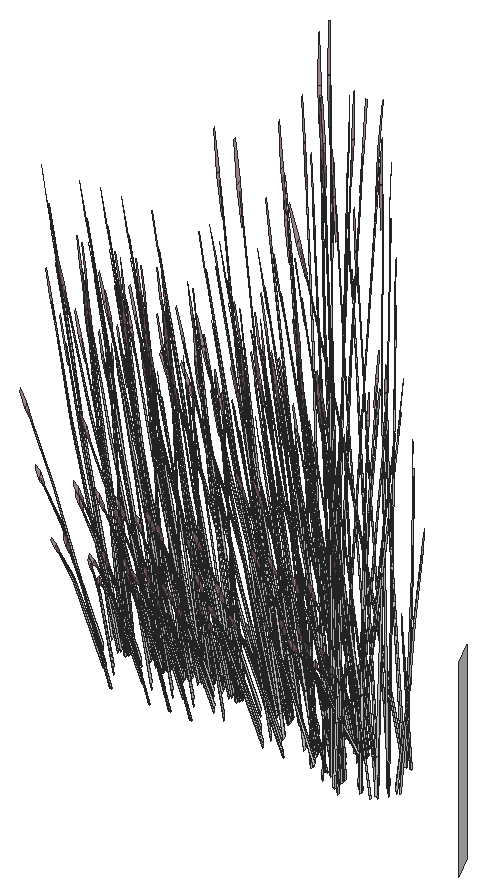
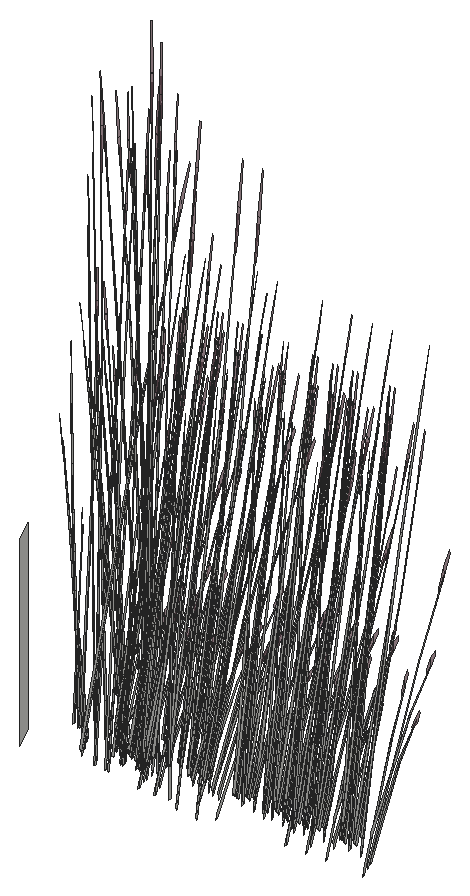
# SketchUp Ruby script. Lengths in inches.
U = 1.inch
M = Sketchup.active_model
def pt(a) = Geom::Point3d.new(a.map { |v| v * U })
def face(e, loops, mat)
  f = e.add_face(loops[0].map { |a| pt(a) })
  loops[1..].each { |l| e.add_face(l.map { |a| pt(a) }).erase! }
  f.material = f.back_material = mat if mat
  f
end
# faces: each face lists its corners as indices into pts; further lists are holes
def faces(e, pts, list, mat = nil) = list.each { |f| face(e, (f[0].is_a?(Array) ? f : [f]).map { |l| l.map { |i| pts[i] } }, mat) }
# xy, xz, yz: faces in a plane at the given z, y or x. An outline is a flat list of corners, or four numbers for a rectangle; further outlines are holes
def ring(l) = l.size == 4 ? [[l[0], l[1]], [l[2], l[1]], [l[2], l[3]], [l[0], l[3]]] : l.each_slice(2).to_a
def flat(e, list, mat, &to3) = list.each { |f| face(e, (f[0].is_a?(Array) ? f : [f]).map { |l| ring(l).map { |u, v| to3.(u, v) } }, mat) }
def xy(e, z, list, mat = nil) = flat(e, list, mat) { |x, y| [x, y, z] }
def xz(e, y, list, mat = nil) = flat(e, list, mat) { |x, z| [x, y, z] }
def yz(e, x, list, mat = nil) = flat(e, list, mat) { |y, z| [x, y, z] }
def lines(e, pts, list) = list.each { |a, b| e.add_line(pt(pts[a]), pt(pts[b])) }
# prism: a flat outline (further loops are holes) pulled along v
def prism(e, loops, v, mat = nil)
  f = face(e, loops, mat); d = Geom::Vector3d.new(v.map { |x| x * U })
  f.pushpull(f.normal.samedirection?(d) ? d.length : -d.length)
end
def box(e, o, s, mat = nil) = prism(e, [[o, [o[0] + s[0], o[1], o[2]], [o[0] + s[0], o[1] + s[1], o[2]], [o[0], o[1] + s[1], o[2]]]], [0, 0, s[2]], mat)
def at(x, y, z, deg = 0) = Geom::Transformation.translation(pt([x, y, z])) * Geom::Transformation.rotation(ORIGIN, Z_AXIS, deg.degrees)
def axes(o, x, y, z) = Geom::Transformation.new([*x, 0, *y, 0, *z, 0, *pt(o).to_a, 1])
def part(name) = M.definitions.add(name)
# library, detail: a bought-in or finely detailed component or shape, given as its bounding box
def library(name, o, s) = part(name).tap { |d| box(d.entities, o, s) }
def detail(e, o, s) = box(e.add_group.entities, o, s)
def put(e, d, t, mat = nil) = e.add_instance(d, t).tap { |i| i.material = mat if mat }
def group(e, t, mat = nil) = e.add_group.tap { |g| g.transformation = t; g.material = mat if mat }.entities
root = M.entities
M.materials.add("LightPink_Translucent").color = [144, 107, 117]
M.materials["LightPink_Translucent"].alpha = 0.75
c1 = part("blade")
p = [[2.15,0.21,22],[0,0.17,0],[0.09,0.45,0],[2.18,0.31,22],[2.29,0.31,22],[0.38,0.45,0],
  [2.48,0.24,33],[2.49,0.24,33],[2.48,0.22,33]]
faces(c1.entities,p,[[0,1,2,3],[4,5,2,3],[6,3,4,7],[8,0,3,6]])
c2 = part("seeds")
p = [[0.3,-0.1,1.38],[-0.01,-0.03,1.59],[-0.01,-0.03,0.03],[0.14,-0.07,-0.07],[0.29,-0.03,3],[0.15,0.01,3.11]]
faces(c2.entities,p,[[0,1,2,3],[1,0,4,5]],"LightPink_Translucent")
c3 = part("blade with seeds")
put(c3.entities,c1,at(0,0,0))
put(c3.entities,c2,axes([2.4,0.25,30.99],[1.5799,-0.05474,1.17369],[-0.12525,1.92788,0.29478],[-0.07173,-0.02425,1.56792]))
p = [[372.76,351.04,618],[373.98,348.58,618],[373.98,348.58,636],[372.76,351.04,636]]
faces(root,p,[[0,1,2,3]])
put(root,c3,axes([358.76,353.51,622.98],[-0.16845,-0.3792,-0.71045],[0.34676,-0.21133,0.08574],[-0.03939,-0.18322,1.00501]))
put(root,c3,axes([337.4375,352.92,620.59],[-0.02137,0.15256,1.43002],[-0.31245,0.12771,-0.30754],[-0.07303,-0.19719,0.61141]))
put(root,c3,axes([360.3,353.52,622.98],[-0.16845,-0.3792,-0.71045],[0.34676,-0.21133,0.08574],[-0.03939,-0.18322,1.00501]))
put(root,c3,axes([364.08,350.79,620.13],[-0.2439,0.26754,-0.03893],[-0.22348,-0.29302,-0.17649],[-0.01573,-0.08303,0.58215]))
put(root,c3,axes([342.99,352.94,620.59],[-0.02137,0.15256,1.43002],[-0.31245,0.12771,-0.30754],[-0.07303,-0.19719,0.61141]))
put(root,c3,axes([353.66,352.8,622.68],[-0.34695,-0.11691,-0.51099],[0.11892,-0.40083,-0.3958],[-0.03181,-0.16138,0.97773]))
put(root,c3,axes([353.87,351.8,620.77],[0.04528,0.27194,1.1486],[-0.25117,-0.15062,0.84392],[0.02703,-0.13924,0.25299]))
put(root,c3,axes([341.92,352.51,619.49],[-0.0592,0.0168,1.76342],[-0.32738,-0.18913,-0.26939],[0.00549,-0.15776,0.30037]))
put(root,c3,axes([345.83,352.52,619.49],[-0.0592,0.0168,1.76342],[-0.32738,-0.18913,-0.26939],[0.00549,-0.15776,0.30037]))
put(root,c3,axes([360.47,351.21,620.43],[0.39767,0.22603,0.24065],[-0.19139,0.46966,0.50002],[0,-0.10827,1.60543]))
put(root,c3,axes([357.66,353,620.59],[-0.02137,0.15256,1.43002],[-0.31245,0.12771,-0.30754],[-0.07303,-0.19719,0.61141]))
put(root,c3,axes([350.43,352.81,622.72],[-0.00341,-0.09282,1.74944],[-0.28775,-0.26825,-0.27667],[0.04449,-0.16261,0.14031]))
put(root,c3,axes([349.22,352.79,622.53],[0.1064,-0.35863,-0.35414],[0.31043,0.1046,0.4572],[-0.02846,-0.14439,0.87481]))
put(root,c3,axes([360.32,351.84,620.4375],[0.09355,-0.55261,-0.23429],[0.44354,0.09633,0.51271],[-0.0775,-0.07631,1.5644]))
put(root,c3,axes([349.46,353.26,621.875],[-0.06572,0.16029,1.71376],[-0.27569,-0.33172,0.13857],[0.12437,-0.20675,0.73262]))
put(root,c3,axes([359.2,353.01,620.59],[-0.02137,0.15256,1.43002],[-0.31245,0.12771,-0.30754],[-0.07303,-0.19719,0.61141]))
put(root,c3,axes([350.35,352.47,622.71],[-0.03584,0.03562,1.77383],[-0.35118,-0.12018,-0.16761],[-0.01271,-0.15545,0.31391]))
put(root,c3,axes([355.12,352.28,623.09],[0.39316,-0.11987,0.53763],[0.06823,0.47021,0.4433],[-0.09247,-0.13858,1.11249]))
put(root,c3,axes([354.41,353.1,622.68],[-0.25266,-0.31335,-0.51099],[0.2669,-0.27442,-0.3958],[0.03844,-0.15921,0.97773]))
put(root,c3,axes([338.24,352.59,619.49],[-0.0592,0.0168,1.76342],[-0.32738,-0.18913,-0.26939],[0.00549,-0.15776,0.30037]))
put(root,c3,axes([359.33,350.21,622.68],[-0.25628,0.30892,-0.51099],[-0.22444,-0.32634,-0.3958],[-0.13021,-0.047,0.97773]))
put(root,c3,axes([343.79,352.61,619.49],[-0.0592,0.0168,1.76342],[-0.32738,-0.18913,-0.26939],[0.00549,-0.15776,0.30037]))
put(root,c3,axes([362.875,350.92,622.72],[-0.07594,-0.00329,1.74944],[-0.24177,0.32918,-0.27667],[-0.129,-0.06726,0.14031]))
put(root,c3,axes([365.74,352.56,623.03],[-0.32648,-0.25715,-0.1216],[0.18809,-0.3724,-0.67495],[0.09224,-0.12945,1.02557]))
put(root,c3,axes([356.01,352.36,622.73],[0.34777,0.12192,0.48003],[-0.11892,0.40083,0.3958],[-0.0209,-0.15763,0.9933]))
put(root,c3,axes([359.52,350.07,623.05],[0.20082,0.29199,0.35414],[-0.2293,0.2764,-0.4572],[-0.1165,-0.04206,0.87481]))
put(root,c3,axes([358.47,352.66,619.49],[-0.0592,0.0168,1.76342],[-0.32738,-0.18913,-0.26939],[0.00549,-0.15776,0.30037]))
put(root,c3,axes([342.91,353.72,622.98],[0.00918,-0.43138,-0.71045],[0.38672,0.02897,0.08574],[0.04081,-0.18275,1.00501]))
put(root,c3,axes([356.11,352.51,623.03],[-0.34538,0.21713,-0.1216],[-0.16972,-0.38536,-0.67495],[-0.04557,-0.16239,1.02557]))
put(root,c3,axes([353.04,351.56,622.71],[-0.00658,0.0559,1.77383],[-0.32474,0.20287,-0.16761],[-0.09556,-0.1037,0.31391]))
put(root,c3,axes([360.01,352.68,619.49],[-0.0592,0.0168,1.76342],[-0.32738,-0.18913,-0.26939],[0.00549,-0.15776,0.30037]))
put(root,c3,axes([346.83,353.73,622.98],[0.00918,-0.43138,-0.71045],[0.38672,0.02897,0.08574],[0.04081,-0.18275,1.00501]))
put(root,c3,axes([356.83,352.99,623.03],[-0.3879,-0.02311,-0.1216],[0.0106,-0.43749,-0.67495],[0.02694,-0.1685,1.02557]))
put(root,c3,axes([358.75,350.62,620.77],[0.22533,-0.03337,1.1486],[-0.14293,0.29403,0.84392],[-0.11135,-0.04411,0.25299]))
put(root,c3,axes([356.8,352.71,622.53],[0.23881,-0.24554,-0.35414],[0.22606,0.28036,0.4572],[0.0344,-0.14245,0.87481]))
put(root,c3,axes([354.74,351.85,620.77],[0.18411,0.16231,1.1486],[-0.26813,0.09757,0.84392],[-0.05737,-0.12474,0.25299]))
put(root,c3,axes([356.1,352.33,622.73],[0.26007,-0.1585,0.0643],[0.12729,0.28902,0.50621],[-0.02512,-0.1274,0.77189]))
put(root,c3,axes([349.0625,353.03,622.68],[-0.34695,-0.11691,-0.51099],[0.11892,-0.40083,-0.3958],[-0.03181,-0.16138,0.97773]))
put(root,c3,axes([355.18,352.71,622.98],[-0.30095,-0.22541,-0.71045],[0.21388,-0.395,0.08574],[-0.10904,-0.13459,1.00501]))
put(root,c3,axes([349.28,352.03,620.77],[0.04528,0.27194,1.1486],[-0.25117,-0.15062,0.84392],[0.02703,-0.13924,0.25299]))
put(root,c3,axes([339.23,353.8,622.98],[0.00918,-0.43138,-0.71045],[0.38672,0.02897,0.08574],[0.04081,-0.18275,1.00501]))
put(root,c3,axes([344.78,353.82,622.98],[0.00918,-0.43138,-0.71045],[0.38672,0.02897,0.08574],[0.04081,-0.18275,1.00501]))
put(root,c3,axes([355.08,352.41,622.53],[-0.05451,-0.37564,-0.35414],[0.31161,-0.09919,0.4572],[-0.0837,-0.10765,0.87481]))
put(root,c3,axes([343.45,353.05,622.72],[-0.00341,-0.09282,1.74944],[-0.28775,-0.26825,-0.27667],[0.04449,-0.16261,0.14031]))
put(root,c3,axes([342.24,353.03,622.53],[0.1064,-0.35863,-0.35414],[0.31043,0.1046,0.4572],[-0.02846,-0.14439,0.87481]))
put(root,c3,axes([342.48,353.5,621.875],[-0.06572,0.16029,1.71376],[-0.27569,-0.33172,0.13857],[0.12437,-0.20675,0.73262]))
put(root,c3,axes([347.37,353.06,622.72],[-0.00341,-0.09282,1.74944],[-0.28775,-0.26825,-0.27667],[0.04449,-0.16261,0.14031]))
put(root,c3,axes([343.37,352.71,622.71],[-0.03584,0.03562,1.77383],[-0.35118,-0.12018,-0.16761],[-0.01271,-0.15545,0.31391]))
put(root,c3,axes([346.16,353.04,622.53],[0.1064,-0.35863,-0.35414],[0.31043,0.1046,0.4572],[-0.02846,-0.14439,0.87481]))
put(root,c3,axes([346.39,353.51,621.875],[-0.06572,0.16029,1.71376],[-0.27569,-0.33172,0.13857],[0.12437,-0.20675,0.73262]))
put(root,c3,axes([347.29,352.72,622.71],[-0.03584,0.03562,1.77383],[-0.35118,-0.12018,-0.16761],[-0.01271,-0.15545,0.31391]))
put(root,c3,axes([349.8125,353.34,622.68],[-0.25266,-0.31335,-0.51099],[0.2669,-0.27442,-0.3958],[0.03844,-0.15921,0.97773]))
put(root,c3,axes([359.46,353.875,622.98],[0.00918,-0.43138,-0.71045],[0.38672,0.02897,0.08574],[0.04081,-0.18275,1.00501]))
put(root,c3,axes([360.34,350.89,620.72],[-0.38326,0.02879,0.44739],[-0.03466,-0.47788,-0.21531],[0.06861,-0.04843,1.43643]))
put(root,c3,axes([361,353.89,622.98],[0.00918,-0.43138,-0.71045],[0.38672,0.02897,0.08574],[0.04081,-0.18275,1.00501]))
put(root,c3,axes([352.96,352.55,623.09],[0.39316,-0.11987,0.53763],[0.06823,0.47021,0.4433],[-0.09247,-0.13858,1.11249]))
put(root,c3,axes([364.39,353.96,621.33],[0.305,0.18805,1.51261],[-0.29879,0.40513,0.59816],[-0.13384,-0.24012,1.26806]))
put(root,c3,axes([359.46,349.89,623.03],[-0.0189,0.47427,-0.1216],[-0.35781,-0.01296,-0.67495],[-0.13781,-0.03295,1.02557]))
put(root,c3,axes([359.35,351.24,620.48],[0,0.46636,0.49651],[-0.39487,0,0],[0,-0.10622,1.57504]))
put(root,c3,axes([339.77,353.125,622.72],[-0.00341,-0.09282,1.74944],[-0.28775,-0.26825,-0.27667],[0.04449,-0.16261,0.14031]))
put(root,c3,axes([338.5625,353.11,622.53],[0.1064,-0.35863,-0.35414],[0.31043,0.1046,0.4572],[-0.02846,-0.14439,0.87481]))
put(root,c3,axes([338.8,353.58,621.875],[-0.06572,0.16029,1.71376],[-0.27569,-0.33172,0.13857],[0.12437,-0.20675,0.73262]))
put(root,c3,axes([339.69,352.79,622.71],[-0.03584,0.03562,1.77383],[-0.35118,-0.12018,-0.16761],[-0.01271,-0.15545,0.31391]))
put(root,c3,axes([345.32,353.15,622.72],[-0.00341,-0.09282,1.74944],[-0.28775,-0.26825,-0.27667],[0.04449,-0.16261,0.14031]))
put(root,c3,axes([344.11,353.13,622.53],[0.1064,-0.35863,-0.35414],[0.31043,0.1046,0.4572],[-0.02846,-0.14439,0.87481]))
put(root,c3,axes([344.35,353.6,621.875],[-0.06572,0.16029,1.71376],[-0.27569,-0.33172,0.13857],[0.12437,-0.20675,0.73262]))
put(root,c3,axes([345.24,352.82,622.71],[-0.03584,0.03562,1.77383],[-0.35118,-0.12018,-0.16761],[-0.01271,-0.15545,0.31391]))
put(root,c3,axes([363.75,351.42,623.05],[0.05451,0.37564,0.35414],[-0.31161,0.09919,-0.4572],[-0.0837,-0.10765,0.87481]))
put(root,c3,axes([348.44,351.79,622.71],[-0.00658,0.0559,1.77383],[-0.32474,0.20287,-0.16761],[-0.09556,-0.1037,0.31391]))
put(root,c3,axes([353.85,352.64,622.73],[0.34777,0.12192,0.48003],[-0.11892,0.40083,0.3958],[-0.0209,-0.15763,0.9933]))
put(root,c3,axes([362.14,351.71,623.03],[-0.17758,-0.42229,-0.1216],[0.31518,-0.20752,-0.67495],[0.13282,-0.05572,1.02557]))
put(root,c3,axes([362.125,351.34,622.68],[0.09562,-0.42421,-0.51099],[0.32782,0.1454,-0.3958],[0.13199,-0.0389,0.97773]))
put(root,c3,axes([362.8,352.66,620.02],[0,-0.46636,-0.49651],[0.39487,0,0],[0,-0.10622,1.57504]))
put(root,c3,axes([363.9,351.28,620.02],[0.33032,-0.23318,-0.49651],[0.19744,0.41812,0],[0.07523,-0.05311,1.57504]))
put(root,c3,axes([360,353.2,622.72],[-0.00341,-0.09282,1.74944],[-0.28775,-0.26825,-0.27667],[0.04449,-0.16261,0.14031]))
put(root,c3,axes([361.61,349.62,620.375],[0.22066,-0.46731,0],[0.36918,0.26061,-0.51607],[0.08408,0.05936,1.63711]))
put(root,c3,axes([358.79,353.18,622.53],[0.1064,-0.35863,-0.35414],[0.31043,0.1046,0.4572],[-0.02846,-0.14439,0.87481]))
put(root,c3,axes([353.95,352.78,623.03],[-0.34538,0.21713,-0.1216],[-0.16972,-0.38536,-0.67495],[-0.04557,-0.16239,1.02557]))
put(root,c3,axes([359.03,353.66,621.875],[-0.06572,0.16029,1.71376],[-0.27569,-0.33172,0.13857],[0.12437,-0.20675,0.73262]))
put(root,c3,axes([359.92,352.87,622.71],[-0.03584,0.03562,1.77383],[-0.35118,-0.12018,-0.16761],[-0.01271,-0.15545,0.31391]))
put(root,c3,axes([361.54,353.21,622.72],[-0.00341,-0.09282,1.74944],[-0.28775,-0.26825,-0.27667],[0.04449,-0.16261,0.14031]))
put(root,c3,axes([360.33,353.2,622.53],[0.1064,-0.35863,-0.35414],[0.31043,0.1046,0.4572],[-0.02846,-0.14439,0.87481]))
put(root,c3,axes([360.5625,353.67,621.875],[-0.06572,0.16029,1.71376],[-0.27569,-0.33172,0.13857],[0.12437,-0.20675,0.73262]))
put(root,c3,axes([365.86,352.09,620.59],[-0.12609,-0.01381,1.43002],[-0.12917,-0.37055,-0.30754],[0.1549,-0.10482,0.61141]))
put(root,c3,axes([362.82,351.66,623.09],[0.29147,-0.34417,0.53763],[0.25138,0.3655,0.4433],[-0.13675,-0.06349,1.11249]))
put(root,c3,axes([361.46,352.88,622.71],[-0.03584,0.03562,1.77383],[-0.35118,-0.12018,-0.16761],[-0.01271,-0.15545,0.31391]))
put(root,c3,axes([354.67,353.27,623.03],[-0.3879,-0.02311,-0.1216],[0.0106,-0.43749,-0.67495],[0.02694,-0.1685,1.02557]))
put(root,c3,axes([342.08,353.27,622.68],[-0.34695,-0.11691,-0.51099],[0.11892,-0.40083,-0.3958],[-0.03181,-0.16138,0.97773]))
put(root,c3,axes([366.55,352.44,622.71],[-0.0461,-0.00354,1.77383],[-0.19143,-0.37951,-0.16761],[0.07688,-0.12478,0.31391]))
put(root,c3,axes([359.01,350.54,621.875],[0.14639,-0.01056,1.71376],[-0.09712,0.45778,0.13857],[-0.20862,-0.02831,0.73262]))
put(root,c3,axes([342.3,352.27,620.77],[0.04528,0.27194,1.1486],[-0.25117,-0.15062,0.84392],[0.02703,-0.13924,0.25299]))
put(root,c3,axes([346,353.28,622.68],[-0.34695,-0.11691,-0.51099],[0.11892,-0.40083,-0.3958],[-0.03181,-0.16138,0.97773]))
put(root,c3,axes([354.64,352.99,622.53],[0.23881,-0.24554,-0.35414],[0.22606,0.28036,0.4572],[0.0344,-0.14245,0.87481]))
put(root,c3,axes([360.29,351.62,620.21],[-0.21202,-0.39143,-0.44739],[0.32115,-0.27564,0.21531],[-0.06861,-0.04843,1.43643]))
put(root,c3,axes([360.33,351.0625,620.36],[0.15345,0.52148,0.45755],[-0.43845,0.18134,0.17955],[0.00536,-0.09582,1.58856]))
put(root,c3,axes([352.58,352.125,620.77],[0.18411,0.16231,1.1486],[-0.26813,0.09757,0.84392],[-0.05737,-0.12474,0.25299]))
put(root,c3,axes([346.21,352.28,620.77],[0.04528,0.27194,1.1486],[-0.25117,-0.15062,0.84392],[0.02703,-0.13924,0.25299]))
put(root,c3,axes([353.95,352.61,622.73],[0.26007,-0.1585,0.0643],[0.12729,0.28902,0.50621],[-0.02512,-0.1274,0.77189]))
put(root,c3,axes([353.02,352.98,622.98],[-0.30095,-0.22541,-0.71045],[0.21388,-0.395,0.08574],[-0.10904,-0.13459,1.00501]))
put(root,c3,axes([352.92,352.69,622.53],[-0.05451,-0.37564,-0.35414],[0.31161,-0.09919,0.4572],[-0.0837,-0.10765,0.87481]))
put(root,c3,axes([338.4,353.35,622.68],[-0.34695,-0.11691,-0.51099],[0.11892,-0.40083,-0.3958],[-0.03181,-0.16138,0.97773]))
put(root,c3,axes([342.83,353.58,622.68],[-0.25266,-0.31335,-0.51099],[0.2669,-0.27442,-0.3958],[0.03844,-0.15921,0.97773]))
put(root,c3,axes([338.62,352.35,620.77],[0.04528,0.27194,1.1486],[-0.25117,-0.15062,0.84392],[0.02703,-0.13924,0.25299]))
put(root,c3,axes([346.75,353.59,622.68],[-0.25266,-0.31335,-0.51099],[0.2669,-0.27442,-0.3958],[0.03844,-0.15921,0.97773]))
put(root,c3,axes([348.37,352.78,623.09],[0.39316,-0.11987,0.53763],[0.06823,0.47021,0.4433],[-0.09247,-0.13858,1.11249]))
put(root,c3,axes([343.95,353.375,622.68],[-0.34695,-0.11691,-0.51099],[0.11892,-0.40083,-0.3958],[-0.03181,-0.16138,0.97773]))
put(root,c3,axes([344.17,352.37,620.77],[0.04528,0.27194,1.1486],[-0.25117,-0.15062,0.84392],[0.02703,-0.13924,0.25299]))
put(root,c3,axes([364.29,352.24,620.06],[0.23773,-0.35053,-0.62353],[0.29532,0.31785,-0.16365],[0.09526,-0.08744,1.37633]))
put(root,c3,axes([362.48,351.46,619.98],[-0.22732,0.05597,1.41583],[-0.03618,-0.44548,0.08104],[0.15921,-0.06743,0.80566]))
put(root,c3,axes([362.89,351.07,620.26],[-0.21881,-0.29821,-0.06488],[0.23965,-0.27324,-0.29416],[0.0679,-0.01924,0.97024]))
put(root,c3,axes([366,351.4,620.77],[-0.11756,0.2374,1.1486],[-0.10105,-0.31895,0.84392],[0.09709,-0.07992,0.25299]))
put(root,c3,axes([358.63,353.43,622.68],[-0.34695,-0.11691,-0.51099],[0.11892,-0.40083,-0.3958],[-0.03181,-0.16138,0.97773]))
put(root,c3,axes([339.15,353.66,622.68],[-0.25266,-0.31335,-0.51099],[0.2669,-0.27442,-0.3958],[0.03844,-0.15921,0.97773]))
put(root,c3,axes([358.85,352.43,620.77],[0.04528,0.27194,1.1486],[-0.25117,-0.15062,0.84392],[0.02703,-0.13924,0.25299]))
put(root,c3,axes([355.21,352.38,622.73],[0.16041,-0.29625,0.0643],[0.22843,0.17248,0.50621],[-0.07385,-0.09498,0.77189]))
put(root,c3,axes([360.17,353.44,622.68],[-0.34695,-0.11691,-0.51099],[0.11892,-0.40083,-0.3958],[-0.03181,-0.16138,0.97773]))
put(root,c3,axes([354.59,352.34,619.49],[-0.03419,0.06144,1.76342],[-0.3455,0.13246,-0.26939],[-0.08346,-0.12049,0.30037]))
put(root,c3,axes([349.26,352.87,622.73],[0.34777,0.12192,0.48003],[-0.11892,0.40083,0.3958],[-0.0209,-0.15763,0.9933]))
put(root,c3,axes([341.46,352.03,622.71],[-0.00658,0.0559,1.77383],[-0.32474,0.20287,-0.16761],[-0.09556,-0.1037,0.31391]))
put(root,c3,axes([360.38,352.4375,620.77],[0.04528,0.27194,1.1486],[-0.25117,-0.15062,0.84392],[0.02703,-0.13924,0.25299]))
put(root,c3,axes([360.25,351.47,620.72],[-0.17124,0.42022,0.44739],[-0.35581,-0.20224,-0.21531],[0,-0.09687,1.43643]))
put(root,c3,axes([345.38,352.04,622.71],[-0.00658,0.0559,1.77383],[-0.32474,0.20287,-0.16761],[-0.09556,-0.1037,0.31391]))
put(root,c3,axes([344.7,353.68,622.68],[-0.25266,-0.31335,-0.51099],[0.2669,-0.27442,-0.3958],[0.03844,-0.15921,0.97773]))
put(root,c3,axes([349.36,353.02,623.03],[-0.34538,0.21713,-0.1216],[-0.16972,-0.38536,-0.67495],[-0.04557,-0.16239,1.02557]))
put(root,c3,axes([350.08,353.5,623.03],[-0.3879,-0.02311,-0.1216],[0.0106,-0.43749,-0.67495],[0.02694,-0.1685,1.02557]))
put(root,c3,axes([360.88,351.11,620.21],[0,-0.53961,0],[0.44133,0,0],[0,0,1.79456]))
put(root,c3,axes([359.38,353.73,622.68],[-0.25266,-0.31335,-0.51099],[0.2669,-0.27442,-0.3958],[0.03844,-0.15921,0.97773]))
put(root,c3,axes([350.05,353.22,622.53],[0.23881,-0.24554,-0.35414],[0.22606,0.28036,0.4572],[0.0344,-0.14245,0.87481]))
put(root,c3,axes([347.99,352.36,620.77],[0.18411,0.16231,1.1486],[-0.26813,0.09757,0.84392],[-0.05737,-0.12474,0.25299]))
put(root,c3,axes([360.92,353.74,622.68],[-0.25266,-0.31335,-0.51099],[0.2669,-0.27442,-0.3958],[0.03844,-0.15921,0.97773]))
put(root,c3,axes([337.78,352.11,622.71],[-0.00658,0.0559,1.77383],[-0.32474,0.20287,-0.16761],[-0.09556,-0.1037,0.31391]))
put(root,c3,axes([349.35,352.84,622.73],[0.26007,-0.1585,0.0643],[0.12729,0.28902,0.50621],[-0.02512,-0.1274,0.77189]))
put(root,c3,axes([355.16,354.03,620.1],[-0.14494,-0.47823,-0.69835],[0.41752,-0.17223,-0.18329],[-0.01602,-0.16194,1.54149]))
put(root,c3,axes([348.43,353.22,622.98],[-0.30095,-0.22541,-0.71045],[0.21388,-0.395,0.08574],[-0.10904,-0.13459,1.00501]))
put(root,c3,axes([343.33,352.13,622.71],[-0.00658,0.0559,1.77383],[-0.32474,0.20287,-0.16761],[-0.09556,-0.1037,0.31391]))
put(root,c3,axes([354.41,352.96,621.875],[0.1311,0.08035,1.71376],[-0.27131,0.33708,0.13857],[-0.16909,-0.15206,0.73262]))
put(root,c3,axes([361.42,349.86,620.48],[-0.33032,-0.23318,0.49651],[0.19744,-0.41812,0],[0.07523,0.05311,1.57504]))
put(root,c3,axes([348.33,352.92,622.53],[-0.05451,-0.37564,-0.35414],[0.31161,-0.09919,0.4572],[-0.0837,-0.10765,0.87481]))
put(root,c3,axes([357.1,352.57,619.49],[-0.05283,-0.03674,1.76342],[-0.13569,-0.41045,-0.26939],[0.09154,-0.11138,0.30037]))
put(root,c3,axes([362.0625,351.5,622.98],[0.31014,-0.20596,-0.71045],[0.17284,0.42397,0.08574],[0.14985,-0.04816,1.00501]))
put(root,c3,axes([365.83,352.3,622.53],[0.30722,-0.06665,-0.35414],[0.08112,0.381,0.4572],[0.08804,-0.10234,0.87481]))
put(root,c3,axes([358.01,352.1875,622.71],[-0.00658,0.0559,1.77383],[-0.32474,0.20287,-0.16761],[-0.09556,-0.1037,0.31391]))
put(root,c3,axes([341.39,353.02,623.09],[0.39316,-0.11987,0.53763],[0.06823,0.47021,0.4433],[-0.09247,-0.13858,1.11249]))
put(root,c3,axes([359.55,352.2,622.71],[-0.00658,0.0559,1.77383],[-0.32474,0.20287,-0.16761],[-0.09556,-0.1037,0.31391]))
put(root,c3,axes([345.31,353.03,623.09],[0.39316,-0.11987,0.53763],[0.06823,0.47021,0.4433],[-0.09247,-0.13858,1.11249]))
put(root,c3,axes([362.95,351.66,622.73],[0.01777,-0.35463,0.0643],[0.26836,0.00972,0.50621],[-0.1028,-0.03711,0.77189]))
put(root,c3,axes([342.28,353.11,622.73],[0.34777,0.12192,0.48003],[-0.11892,0.40083,0.3958],[-0.0209,-0.15763,0.9933]))
put(root,c3,axes([337.71,353.1,623.09],[0.39316,-0.11987,0.53763],[0.06823,0.47021,0.4433],[-0.09247,-0.13858,1.11249]))
put(root,c3,axes([360.1,351.77,620.06],[-0.36714,-0.07646,-0.62353],[0.07747,-0.47163,-0.16365],[-0.10956,-0.05715,1.37633]))
put(root,c3,axes([346.2,353.12,622.73],[0.34777,0.12192,0.48003],[-0.11892,0.40083,0.3958],[-0.0209,-0.15763,0.9933]))
put(root,c3,axes([363.875,352.85,620.21],[0.17124,-0.42022,-0.44739],[0.35581,0.20224,0.21531],[0,-0.09687,1.43643]))
put(root,c3,axes([362.85,351.77,622.53],[-0.20082,-0.29199,-0.35414],[0.2293,-0.2764,0.4572],[-0.1165,-0.04206,0.87481]))
put(root,c3,axes([360.67,350.77,620.36],[-0.29264,0.42323,0.45755],[-0.34767,-0.3736,0.17955],[0.07055,-0.04224,1.58856]))
put(root,c3,axes([343.26,353.125,623.09],[0.39316,-0.11987,0.53763],[0.06823,0.47021,0.4433],[-0.09247,-0.13858,1.11249]))
put(root,c3,axes([356.01,352.66,623.05],[-0.1064,0.35863,0.35414],[-0.31043,-0.1046,-0.4572],[-0.02846,-0.14439,0.87481]))
put(root,c3,axes([353.06,352.65,622.73],[0.16041,-0.29625,0.0643],[0.22843,0.17248,0.50621],[-0.07385,-0.09498,0.77189]))
put(root,c3,axes([352.43,352.61,619.49],[-0.03419,0.06144,1.76342],[-0.3455,0.13246,-0.26939],[-0.08346,-0.12049,0.30037]))
put(root,c3,axes([342.38,353.26,623.03],[-0.34538,0.21713,-0.1216],[-0.16972,-0.38536,-0.67495],[-0.04557,-0.16239,1.02557]))
put(root,c3,axes([346.3,353.27,623.03],[-0.34538,0.21713,-0.1216],[-0.16972,-0.38536,-0.67495],[-0.04557,-0.16239,1.02557]))
put(root,c3,axes([343.1,353.74,623.03],[-0.3879,-0.02311,-0.1216],[0.0106,-0.43749,-0.67495],[0.02694,-0.1685,1.02557]))
put(root,c3,axes([347.01,353.75,623.03],[-0.3879,-0.02311,-0.1216],[0.0106,-0.43749,-0.67495],[0.02694,-0.1685,1.02557]))
put(root,c3,axes([364.03,352.64,620.67],[-0.04113,-0.53214,-0.29095],[0.42835,-0.03218,-0.50002],[0.07543,-0.07088,1.59708]))
put(root,c3,axes([343.07,353.46,622.53],[0.23881,-0.24554,-0.35414],[0.22606,0.28036,0.4572],[0.0344,-0.14245,0.87481]))
put(root,c3,axes([357.94,353.18,623.09],[0.39316,-0.11987,0.53763],[0.06823,0.47021,0.4433],[-0.09247,-0.13858,1.11249]))
put(root,c3,axes([341.01,352.6,620.77],[0.18411,0.16231,1.1486],[-0.26813,0.09757,0.84392],[-0.05737,-0.12474,0.25299]))
put(root,c3,axes([338.6,353.19,622.73],[0.34777,0.12192,0.48003],[-0.11892,0.40083,0.3958],[-0.0209,-0.15763,0.9933]))
put(root,c3,axes([346.99,353.47,622.53],[0.23881,-0.24554,-0.35414],[0.22606,0.28036,0.4572],[0.0344,-0.14245,0.87481]))
put(root,c3,axes([344.92,352.61,620.77],[0.18411,0.16231,1.1486],[-0.26813,0.09757,0.84392],[-0.05737,-0.12474,0.25299]))
put(root,c3,axes([359.48,353.19,623.09],[0.39316,-0.11987,0.53763],[0.06823,0.47021,0.4433],[-0.09247,-0.13858,1.11249]))
put(root,c3,axes([342.37,353.08,622.73],[0.26007,-0.1585,0.0643],[0.12729,0.28902,0.50621],[-0.02512,-0.1274,0.77189]))
put(root,c3,axes([360.99,351.53,620.3],[-0.32829,-0.4014,-0.06131],[0.32849,-0.40164,0],[-0.01146,-0.01402,1.75571]))
put(root,c3,axes([362.97,352.67,620.03],[0.24637,-0.29097,-0.30978],[0.24637,0.29097,0.30978],[0,-0.09372,1.38974]))
put(root,c3,axes([341.45,353.46,622.98],[-0.30095,-0.22541,-0.71045],[0.21388,-0.395,0.08574],[-0.10904,-0.13459,1.00501]))
put(root,c3,axes([346.29,353.09,622.73],[0.26007,-0.1585,0.0643],[0.12729,0.28902,0.50621],[-0.02512,-0.1274,0.77189]))
put(root,c3,axes([355.04,352.72,622.68],[-0.34827,0.11086,-0.51099],[-0.06092,-0.41983,-0.3958],[-0.09354,-0.12031,0.97773]))
put(root,c3,axes([344.15,353.21,622.73],[0.34777,0.12192,0.48003],[-0.11892,0.40083,0.3958],[-0.0209,-0.15763,0.9933]))
put(root,c3,axes([356.8,352.81,622.73],[0.25132,0.3182,0.48003],[-0.2669,0.27442,0.3958],[0.04636,-0.14929,0.9933]))
put(root,c3,axes([345.37,353.47,622.98],[-0.30095,-0.22541,-0.71045],[0.21388,-0.395,0.08574],[-0.10904,-0.13459,1.00501]))
put(root,c3,axes([338.7,353.33,623.03],[-0.34538,0.21713,-0.1216],[-0.16972,-0.38536,-0.67495],[-0.04557,-0.16239,1.02557]))
put(root,c3,axes([353,354.3,620.1],[-0.14494,-0.47823,-0.69835],[0.41752,-0.17223,-0.18329],[-0.01602,-0.16194,1.54149]))
put(root,c3,axes([339.42,353.82,623.03],[-0.3879,-0.02311,-0.1216],[0.0106,-0.43749,-0.67495],[0.02694,-0.1685,1.02557]))
put(root,c3,axes([341.35,353.16,622.53],[-0.05451,-0.37564,-0.35414],[0.31161,-0.09919,0.4572],[-0.0837,-0.10765,0.87481]))
put(root,c3,axes([344.25,353.36,623.03],[-0.34538,0.21713,-0.1216],[-0.16972,-0.38536,-0.67495],[-0.04557,-0.16239,1.02557]))
put(root,c3,axes([355.28,352.35,623.43],[-0.23555,0.44708,-0.13619],[-0.34112,-0.25757,-0.75594],[-0.11858,-0.12631,1.14864]))
put(root,c3,axes([345.26,353.17,622.53],[-0.05451,-0.37564,-0.35414],[0.31161,-0.09919,0.4572],[-0.0837,-0.10765,0.87481]))
put(root,c3,axes([356.89,352.84,622.73],[0.29004,0.02173,0.0643],[-0.00795,0.32812,0.50621],[0.03035,-0.12569,0.77189]))
put(root,c3,axes([352.25,353.23,621.875],[0.1311,0.08035,1.71376],[-0.27131,0.33708,0.13857],[-0.16909,-0.15206,0.73262]))
put(root,c3,axes([339.39,353.54,622.53],[0.23881,-0.24554,-0.35414],[0.22606,0.28036,0.4572],[0.0344,-0.14245,0.87481]))
put(root,c3,axes([344.97,353.84,623.03],[-0.3879,-0.02311,-0.1216],[0.0106,-0.43749,-0.67495],[0.02694,-0.1685,1.02557]))
put(root,c3,axes([358.83,353.27,622.73],[0.34777,0.12192,0.48003],[-0.11892,0.40083,0.3958],[-0.0209,-0.15763,0.9933]))
put(root,c3,axes([360.16,350.07,620.47],[-0.10196,0.46348,0.17642],[-0.3731,-0.13116,0.35086],[0.06445,-0.00226,1.60407]))
put(root,c3,axes([337.33,352.68,620.77],[0.18411,0.16231,1.1486],[-0.26813,0.09757,0.84392],[-0.05737,-0.12474,0.25299]))
put(root,c3,axes([362.87,351.28,620.13],[-0.10181,0.3808,-0.03893],[-0.31336,-0.11714,-0.17649],[-0.04758,-0.06228,0.58215]))
put(root,c3,axes([362.02,351.58,623.05],[-0.29332,-0.1301,0.35414],[0.08555,-0.37955,-0.4572],[0.11809,-0.0348,0.87481]))
